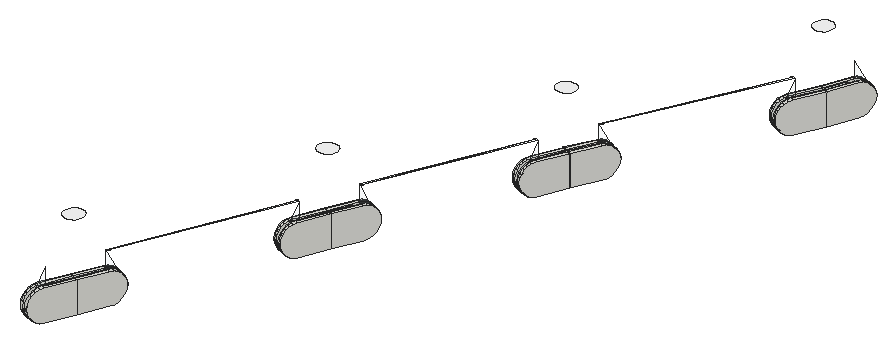
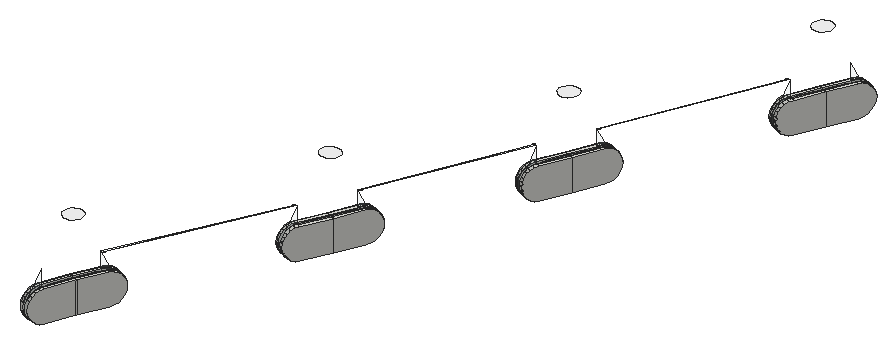
# SketchUp Ruby script. Lengths in inches.
U = 1.inch
M = Sketchup.active_model
def pt(a) = Geom::Point3d.new(a.map { |v| v * U })
def face(e, loops, mat)
  f = e.add_face(loops[0].map { |a| pt(a) })
  loops[1..].each { |l| e.add_face(l.map { |a| pt(a) }).erase! }
  f.material = f.back_material = mat if mat
  f
end
# faces: each face lists its corners as indices into pts; further lists are holes
def faces(e, pts, list, mat = nil) = list.each { |f| face(e, (f[0].is_a?(Array) ? f : [f]).map { |l| l.map { |i| pts[i] } }, mat) }
# xy, xz, yz: faces in a plane at the given z, y or x. An outline is a flat list of corners, or four numbers for a rectangle; further outlines are holes
def ring(l) = l.size == 4 ? [[l[0], l[1]], [l[2], l[1]], [l[2], l[3]], [l[0], l[3]]] : l.each_slice(2).to_a
def flat(e, list, mat, &to3) = list.each { |f| face(e, (f[0].is_a?(Array) ? f : [f]).map { |l| ring(l).map { |u, v| to3.(u, v) } }, mat) }
def xy(e, z, list, mat = nil) = flat(e, list, mat) { |x, y| [x, y, z] }
def xz(e, y, list, mat = nil) = flat(e, list, mat) { |x, z| [x, y, z] }
def yz(e, x, list, mat = nil) = flat(e, list, mat) { |y, z| [x, y, z] }
def lines(e, pts, list) = list.each { |a, b| e.add_line(pt(pts[a]), pt(pts[b])) }
# prism: a flat outline (further loops are holes) pulled along v
def prism(e, loops, v, mat = nil)
  f = face(e, loops, mat); d = Geom::Vector3d.new(v.map { |x| x * U })
  f.pushpull(f.normal.samedirection?(d) ? d.length : -d.length)
end
def box(e, o, s, mat = nil) = prism(e, [[o, [o[0] + s[0], o[1], o[2]], [o[0] + s[0], o[1] + s[1], o[2]], [o[0], o[1] + s[1], o[2]]]], [0, 0, s[2]], mat)
def at(x, y, z, deg = 0) = Geom::Transformation.translation(pt([x, y, z])) * Geom::Transformation.rotation(ORIGIN, Z_AXIS, deg.degrees)
def axes(o, x, y, z) = Geom::Transformation.new([*x, 0, *y, 0, *z, 0, *pt(o).to_a, 1])
def part(name) = M.definitions.add(name)
# library, detail: a bought-in or finely detailed component or shape, given as its bounding box
def library(name, o, s) = part(name).tap { |d| box(d.entities, o, s) }
def detail(e, o, s) = box(e.add_group.entities, o, s)
def put(e, d, t, mat = nil) = e.add_instance(d, t).tap { |i| i.material = mat if mat }
def group(e, t, mat = nil) = e.add_group.tap { |g| g.transformation = t; g.material = mat if mat }.entities
root = M.entities
M.materials.add("Glass_Safety_01").color = [204, 235, 244]
M.materials["Glass_Safety_01"].alpha = 0.1
M.materials.add("[Color_000]").color = [255, 255, 255]
xy(root,351.283,[[864.446,583.7,864.194,583.81,864.292,584.037,864.98,585.615,865.232,585.505],[864.013,583.889,863.761,583.999,864.547,585.803,864.799,585.693,864.112,584.115],[865.232,585.505,864.98,585.615,865.766,587.42,866.018,587.309],[864.799,585.693,864.547,585.803,865.333,587.608,865.585,587.498],[870.556,597.727,870.303,597.837,870.404,598.069,871.089,599.642,871.341,599.53],
  [870.122,597.916,869.87,598.026,870.656,599.83,870.908,599.72,870.224,598.148],[871.341,599.53,871.089,599.642,871.342,599.532],[871.342,599.532,871.089,599.642,871.885,601.441,872.137,601.33],[870.908,599.72,870.656,599.832,871.453,601.633,871.705,601.521],[876.349,610.851,876.097,610.963,876.207,611.21,876.893,612.761,877.142,612.643],
  [875.917,611.043,875.665,611.154,876.462,612.954,876.714,612.843,876.027,611.29],[877.142,612.643,876.893,612.761,876.894,612.763,877.146,612.652,877.144,612.647],[877.146,612.652,876.894,612.763,877.734,614.541,877.983,614.423],[876.715,612.845,876.466,612.963,877.307,614.743,877.556,614.625],[882.822,624.661,882.573,624.779,882.681,625.009,883.414,626.559,883.663,626.441],
  [882.395,624.863,882.145,624.981,882.977,626.738,883.233,626.637,882.503,625.093],[883.672,626.464,883.416,626.565,884.14,628.396,884.396,628.294],[883.233,626.637,882.977,626.738,882.981,626.75,882.986,626.761,883.236,626.643],[883.236,626.643,882.986,626.761,883.7,628.569,883.957,628.468]])
xy(root,351.362,[[864.351,584.171,864.17,584.25,864.799,585.693,864.98,585.615],[864.98,585.615,864.799,585.693,865.428,587.137,865.609,587.059],[870.46,598.198,870.28,598.277,870.908,599.72,870.999,599.681,871.089,599.642],[871.089,599.642,870.999,599.681,870.908,599.72,871.546,601.161,871.726,601.081],[876.257,611.323,876.077,611.403,876.714,612.843,876.804,612.803,876.893,612.761],
  [876.893,612.761,876.804,612.803,876.894,612.763,876.893,612.762],[876.894,612.763,876.804,612.803,876.715,612.845,877.388,614.269,877.566,614.185],[882.741,625.135,882.563,625.219,883.233,626.637,883.325,626.601,883.414,626.559],[883.416,626.565,883.325,626.601,883.236,626.643,883.812,628.102,883.995,628.029],[883.325,626.601,883.233,626.637,883.234,626.64,883.236,626.643]],"Glass_Safety_01")
xy(root,353.33,[[864.351,584.171,864.98,585.615,864.799,585.693,864.17,584.25],[864.98,585.615,865.609,587.059,865.428,587.137,864.799,585.693],[870.46,598.198,871.089,599.642,870.999,599.681,870.908,599.72,870.28,598.277],[871.089,599.642,871.726,601.081,871.546,601.161,870.908,599.72,870.999,599.681],[876.257,611.323,876.893,612.761,876.804,612.803,876.714,612.843,876.077,611.403],
  [876.893,612.761,876.893,612.762,876.894,612.763,876.804,612.803],[876.894,612.763,877.566,614.185,877.388,614.269,876.715,612.845,876.804,612.803],[882.741,625.135,883.414,626.559,883.325,626.601,883.233,626.637,882.563,625.219],[883.416,626.565,883.995,628.029,883.812,628.102,883.236,626.643,883.325,626.601],[883.325,626.601,883.236,626.643,883.234,626.64,883.233,626.637]],"Glass_Safety_01")
xy(root,353.409,[[864.446,583.7,865.232,585.505,864.98,585.615,864.292,584.037,864.194,583.81],[864.013,583.889,864.112,584.115,864.799,585.693,864.547,585.803,863.761,583.999],[865.232,585.505,866.018,587.309,865.766,587.42,864.98,585.615],[864.799,585.693,865.585,587.498,865.333,587.608,864.547,585.803],[870.556,597.727,871.341,599.53,871.089,599.642,870.404,598.069,870.303,597.837],
  [870.122,597.916,870.224,598.148,870.908,599.72,870.656,599.83,869.87,598.026],[871.341,599.53,871.342,599.532,871.089,599.642],[871.342,599.532,872.137,601.33,871.885,601.441,871.089,599.642],[870.908,599.72,871.705,601.521,871.453,601.633,870.656,599.832],[876.349,610.851,877.142,612.643,876.893,612.761,876.207,611.21,876.097,610.963],
  [875.917,611.043,876.027,611.29,876.714,612.843,876.462,612.954,875.665,611.154],[877.142,612.643,877.144,612.647,877.146,612.652,876.894,612.763,876.893,612.761],[877.146,612.652,877.983,614.423,877.734,614.541,876.894,612.763],[876.715,612.845,877.556,614.625,877.307,614.743,876.466,612.963],[882.822,624.661,883.663,626.441,883.414,626.559,882.681,625.009,882.573,624.779],
  [882.395,624.863,882.503,625.093,883.233,626.637,882.977,626.738,882.145,624.981],[883.672,626.464,884.396,628.294,884.14,628.396,883.416,626.565],[883.233,626.637,883.236,626.643,882.986,626.761,882.981,626.75,882.977,626.738],[883.236,626.643,883.957,628.468,883.7,628.569,882.986,626.761]])
xy(root,354.511,[[865.766,587.42,870.224,598.148,865.585,587.498],[865.766,587.42,870.404,598.069,870.224,598.148],[871.885,601.441,876.027,611.29,871.705,601.521],[871.885,601.441,876.207,611.21,876.027,611.29],[877.734,614.541,882.503,625.093,877.556,614.625],
  [877.734,614.541,882.681,625.009,882.503,625.093]],"Glass_Safety_01")
xy(root,357.267,[[864.935,585.026,865.096,585.059,865.243,585.132,865.366,585.242,865.456,585.379,865.508,585.535,865.518,585.699,865.485,585.86,865.411,586.007,865.302,586.13,865.165,586.221,865.009,586.273,864.844,586.282,864.683,586.249,864.536,586.176,864.413,586.066,864.323,585.929,864.271,585.773,864.261,585.609,864.294,585.448,864.368,585.301,864.477,585.178,864.614,585.087,864.77,585.035],[871.044,599.053,871.205,599.086,871.352,599.159,871.475,599.269,871.565,599.406,871.617,599.562,871.627,599.726,871.594,599.887,871.52,600.034,871.411,600.157,871.274,600.248,871.118,600.3,870.954,600.309,870.793,600.276,870.646,600.203,870.523,600.093,870.432,599.956,870.38,599.8,870.37,599.636,870.403,599.475,870.477,599.328,870.586,599.205,870.724,599.114,870.88,599.0625],[876.849,612.175,877.01,612.208,877.157,612.281,877.28,612.391,877.37,612.528,877.422,612.684,877.432,612.848,877.399,613.009,877.325,613.156,877.216,613.279,877.079,613.37,876.923,613.422,876.759,613.431,876.598,613.398,876.451,613.325,876.328,613.215,876.237,613.078,876.185,612.922,876.175,612.758,876.208,612.597,876.282,612.45,876.391,612.327,876.529,612.236,876.685,612.184],[883.37,625.973,883.531,626.006,883.678,626.079,883.801,626.189,883.891,626.326,883.943,626.482,883.953,626.646,883.92,626.807,883.846,626.954,883.737,627.077,883.6,627.168,883.444,627.22,883.28,627.229,883.119,627.196,882.971,627.123,882.849,627.013,882.758,626.876,882.706,626.72,882.696,626.556,882.729,626.395,882.803,626.248,882.912,626.125,883.049,626.034,883.206,625.982]],"[Color_000]")
p = [[865.232,585.505,353.409],[864.446,583.7,353.409],[864.337,583.448,353.373],[864.234,583.213,353.267],[864.146,583.011,353.098],[864.079,582.856,352.877],
  [864.036,582.759,352.621],[864.022,582.725,352.346],[864.036,582.759,352.071],[864.079,582.856,351.815],[864.146,583.011,351.594],[864.234,583.213,351.425],
  [864.337,583.448,351.319],[864.446,583.7,351.283],[865.232,585.505,351.283],[864.013,583.889,351.283],[864.112,584.115,351.283],[864.112,584.115,353.409],
  [864.013,583.889,353.409],[863.903,583.636,353.373],[863.801,583.401,353.267],[863.713,583.199,353.098],[863.646,583.045,352.877],[863.603,582.947,352.621],
  [863.589,582.914,352.346],[863.603,582.947,352.071],[863.646,583.045,351.815],[863.713,583.199,351.594],[863.801,583.401,351.425],[863.903,583.636,351.319],
  [864.292,584.037,353.409],[864.292,584.037,351.283],[864.194,583.81,351.283],[864.084,583.558,351.319],[863.981,583.323,351.425],[863.894,583.121,351.594],
  [863.826,582.966,351.815],[863.784,582.869,352.071],[863.782,582.865,352.098],[864.043,583.463,353.33],[864.084,583.558,353.373],[864.194,583.81,353.409],
  [863.761,583.999,353.409],[864.547,585.803,353.409],[864.547,585.803,351.283],[863.761,583.999,351.283],[863.651,583.746,351.319],[863.548,583.511,351.425],
  [863.46,583.31,351.594],[863.393,583.155,351.815],[863.351,583.057,352.071],[863.336,583.024,352.346],[863.351,583.057,352.621],[863.393,583.155,352.877],
  [863.46,583.31,353.098],[863.548,583.511,353.267],[863.651,583.746,353.373],[864.98,585.615,351.283],[864.98,585.615,353.409],[864.98,585.615,353.33],
  [864.351,584.171,353.33],[864.351,584.171,351.362],[864.98,585.615,351.362],[864.799,585.693,353.409],[864.799,585.693,351.283],[864.799,585.693,351.362],
  [864.17,584.25,351.362],[864.17,584.25,353.33],[864.799,585.693,353.33],[866.018,587.309,353.409],[866.018,587.309,351.283],[866.128,587.562,351.319],
  [866.231,587.797,351.425],[866.319,587.999,351.594],[866.386,588.153,351.815],[866.428,588.251,352.071],[866.443,588.284,352.346],[866.428,588.251,352.621],
  [866.386,588.153,352.877],[866.319,587.999,353.098],[866.231,587.797,353.267],[866.128,587.562,353.373],[865.766,587.42,353.409],[865.766,587.42,351.283],
  [865.609,587.059,351.362],[865.609,587.059,353.33],[865.585,587.498,351.283],[865.585,587.498,353.409],[865.428,587.137,353.33],[865.428,587.137,351.362],
  [865.333,587.608,353.409],[865.442,587.86,353.373],[865.545,588.095,353.267],[865.633,588.297,353.098],[865.7,588.452,352.877],[865.743,588.55,352.621],
  [865.757,588.583,352.346],[865.743,588.55,352.071],[865.7,588.452,351.815],[865.633,588.297,351.594],[865.545,588.095,351.425],[865.442,587.86,351.319],
  [865.333,587.608,351.283],[865.876,587.672,351.319],[865.978,587.907,351.425],[866.066,588.109,351.594],[866.133,588.264,351.815],[866.176,588.361,352.071],
  [866.19,588.394,352.346],[866.176,588.361,352.621],[866.133,588.264,352.877],[866.066,588.109,353.098],[865.978,587.907,353.267],[865.876,587.672,353.373],
  [865.695,587.75,351.319],[865.798,587.985,351.425],[865.885,588.187,351.594],[865.953,588.342,351.815],[865.995,588.439,352.071],[866.01,588.473,352.346],
  [866.003,588.457,352.475],[865.869,588.149,353.13],[865.798,587.985,353.267],[865.695,587.75,353.373],[870.556,597.727,351.283],[871.341,599.53,351.283],
  [871.341,599.53,353.409],[870.556,597.727,353.409],[870.446,597.475,353.373],[870.343,597.24,353.267],[870.255,597.038,353.098],[870.188,596.883,352.877],
  [870.146,596.786,352.621],[870.131,596.752,352.346],[870.146,596.786,352.071],[870.188,596.883,351.815],[870.255,597.038,351.594],[870.343,597.24,351.425],
  [870.446,597.475,351.319],[870.122,597.916,351.283],[870.224,598.148,351.283],[870.224,598.148,353.409],[870.122,597.916,353.409],[870.013,597.663,353.373],
  [869.91,597.428,353.267],[869.822,597.226,353.098],[869.755,597.072,352.877],[869.712,596.974,352.621],[869.698,596.941,352.346],[869.712,596.974,352.071],
  [869.755,597.072,351.815],[869.822,597.226,351.594],[869.91,597.428,351.425],[870.013,597.663,351.319],[870.404,598.069,353.409],[870.404,598.069,351.283],
  [870.303,597.837,351.283],[870.193,597.585,351.319],[870.091,597.35,351.425],[870.003,597.148,351.594],[869.935,596.993,351.815],[869.898,596.906,352.042],
  [870.164,597.519,353.343],[870.193,597.585,353.373],[870.303,597.837,353.409],[869.87,598.026,353.409],[870.656,599.83,353.409],[870.656,599.83,351.283],
  [869.87,598.026,351.283],[869.76,597.773,351.319],[869.658,597.538,351.425],[869.57,597.337,351.594],[869.502,597.182,351.815],[869.46,597.084,352.071],
  [869.445,597.051,352.346],[869.46,597.084,352.621],[869.502,597.182,352.877],[869.57,597.337,353.098],[869.658,597.538,353.267],[869.76,597.773,353.373],
  [870.908,599.72,353.409],[870.908,599.72,351.283],[870.908,599.72,351.362],[870.28,598.277,351.362],[870.28,598.277,353.33],[870.908,599.72,353.33],
  [871.089,599.642,351.283],[871.089,599.642,353.409],[871.089,599.642,353.33],[870.46,598.198,353.33],[870.46,598.198,351.362],[871.089,599.642,351.362],
  [871.342,599.532,353.409],[871.342,599.532,351.283],[872.137,601.33,353.409],[872.137,601.33,351.283],[872.248,601.582,351.319],[872.352,601.816,351.425],
  [872.441,602.017,351.594],[872.51,602.172,351.815],[872.553,602.269,352.071],[872.567,602.302,352.346],[872.553,602.269,352.621],[872.51,602.172,352.877],
  [872.441,602.017,353.098],[872.352,601.816,353.267],[872.248,601.582,353.373],[871.885,601.441,353.409],[871.885,601.441,351.283],[871.726,601.081,351.362],
  [871.726,601.081,353.33],[870.656,599.832,353.409],[870.656,599.832,351.283],[871.705,601.521,351.283],[871.705,601.521,353.409],[871.546,601.161,353.33],
  [871.546,601.161,351.362],[871.453,601.633,353.409],[871.564,601.884,353.373],[871.668,602.119,353.267],[871.757,602.32,353.098],[871.825,602.474,352.877],
  [871.868,602.572,352.621],[871.883,602.605,352.346],[871.868,602.572,352.071],[871.825,602.474,351.815],[871.757,602.32,351.594],[871.668,602.119,351.425],
  [871.564,601.884,351.319],[871.453,601.633,351.283],[871.996,601.693,351.319],[872.1,601.927,351.425],[872.189,602.129,351.594],[872.258,602.283,351.815],
  [872.3,602.38,352.071],[872.315,602.414,352.346],[872.3,602.38,352.621],[872.258,602.283,352.877],[872.189,602.129,353.098],[872.1,601.927,353.267],
  [871.996,601.693,353.373],[871.816,601.773,351.319],[871.92,602.007,351.425],[872.009,602.208,351.594],[872.077,602.363,351.815],[872.12,602.46,352.071],
  [872.132,602.485,352.279],[871.956,602.088,353.199],[871.92,602.007,353.267],[871.816,601.773,353.373],[876.349,610.851,351.283],[877.142,612.643,351.283],
  [877.142,612.643,353.409],[876.349,610.851,353.409],[876.238,610.6,353.373],[876.134,610.365,353.267],[876.045,610.164,353.098],[875.977,610.01,352.877],
  [875.934,609.912,352.621],[875.919,609.879,352.346],[875.934,609.912,352.071],[875.977,610.01,351.814],[876.045,610.164,351.594],[876.134,610.365,351.425],
  [876.238,610.6,351.319],[876.207,611.21,353.409],[876.893,612.761,353.409],[876.893,612.761,353.33],[876.893,612.761,351.362],[876.893,612.761,351.283],
  [876.207,611.21,351.283],[876.097,610.963,351.283],[875.986,610.711,351.319],[875.882,610.477,351.425],[875.793,610.276,351.594],[875.725,610.121,351.814],
  [875.709,610.086,351.908],[875.682,610.024,352.071],[875.667,609.991,352.346],[875.682,610.024,352.621],[875.725,610.121,352.877],[875.793,610.276,353.098],
  [875.882,610.477,353.267],[875.986,610.711,353.373],[875.989,610.719,353.374],[876.097,610.963,353.409],[875.917,611.043,351.283],[876.027,611.29,351.283],
  [876.027,611.29,353.409],[875.917,611.043,353.409],[875.806,610.791,353.373],[875.702,610.557,353.267],[875.613,610.355,353.098],[875.545,610.201,352.877],
  [875.502,610.104,352.621],[875.487,610.07,352.346],[875.502,610.104,352.071],[875.545,610.201,351.814],[875.613,610.355,351.594],[875.702,610.557,351.425],
  [875.806,610.791,351.319],[875.665,611.154,353.409],[876.462,612.954,353.409],[876.462,612.954,351.283],[875.665,611.154,351.283],[875.554,610.902,351.319],
  [875.45,610.668,351.425],[875.361,610.467,351.594],[875.293,610.312,351.814],[875.25,610.215,352.071],[875.235,610.182,352.346],[875.25,610.215,352.621],
  [875.293,610.312,352.877],[875.361,610.467,353.098],[875.45,610.668,353.267],[875.554,610.902,353.373],[876.714,612.843,353.409],[876.714,612.843,351.283],
  [876.714,612.843,351.362],[876.077,611.403,351.362],[876.077,611.403,353.33],[876.714,612.843,353.33],[877.144,612.647,353.409],[877.144,612.647,351.283],
  [877.146,612.652,351.283],[877.146,612.652,353.409],[877.983,614.423,351.283],[878.101,614.672,351.319],[878.21,614.903,351.425],[878.304,615.103,351.594],
  [878.376,615.255,351.814],[878.422,615.351,352.071],[878.437,615.384,352.346],[878.422,615.351,352.621],[878.376,615.255,352.877],[878.304,615.103,353.098],
  [878.21,614.903,353.267],[878.101,614.672,353.373],[877.983,614.423,353.409],[876.894,612.763,351.283],[876.894,612.763,351.362],[876.894,612.763,353.33],
  [876.894,612.763,353.409],[876.715,612.845,351.283],[876.715,612.845,351.362],[876.715,612.845,353.33],[876.715,612.845,353.409],[876.466,612.963,353.409],
  [876.466,612.963,351.283],[877.556,614.625,351.283],[877.556,614.625,353.409],[877.388,614.269,353.33],[877.388,614.269,351.362],[877.734,614.541,353.409],
  [877.851,614.789,353.373],[877.961,615.021,353.267],[878.055,615.22,353.098],[878.127,615.373,352.877],[878.173,615.469,352.621],[878.188,615.502,352.346],
  [878.173,615.469,352.071],[878.127,615.373,351.814],[878.055,615.22,351.594],[877.961,615.021,351.425],[877.851,614.789,351.319],[877.734,614.541,351.283],
  [877.307,614.743,353.409],[877.424,614.991,353.373],[877.534,615.223,353.267],[877.628,615.422,353.098],[877.7,615.575,352.877],[877.745,615.671,352.621],
  [877.761,615.704,352.346],[877.745,615.671,352.071],[877.7,615.575,351.814],[877.628,615.422,351.594],[877.534,615.223,351.425],[877.424,614.991,351.319],
  [877.307,614.743,351.283],[877.673,614.874,351.319],[877.783,615.105,351.425],[877.877,615.304,351.594],[877.949,615.457,351.814],[877.995,615.553,352.071],
  [878.01,615.586,352.346],[878.003,615.572,352.466],[877.857,615.263,353.133],[877.783,615.105,353.267],[877.673,614.874,353.373],[883.663,626.441,353.409],
  [882.822,624.661,353.409],[882.704,624.413,353.373],[882.595,624.181,353.267],[882.501,623.982,353.098],[882.428,623.829,352.877],[882.383,623.733,352.621],
  [882.367,623.7,352.346],[882.383,623.733,352.071],[882.428,623.829,351.814],[882.501,623.982,351.594],[882.595,624.181,351.425],[882.704,624.413,351.319],
  [882.822,624.661,351.283],[883.663,626.441,351.283],[882.503,625.093,353.409],[882.503,625.093,351.283],[882.395,624.863,351.283],[882.277,624.615,351.319],
  [882.167,624.383,351.425],[882.073,624.184,351.594],[882.001,624.031,351.814],[881.956,623.935,352.071],[881.94,623.902,352.346],[881.956,623.935,352.621],
  [882.001,624.031,352.877],[882.073,624.184,353.098],[882.167,624.383,353.267],[882.277,624.615,353.373],[882.395,624.863,353.409],[883.233,626.637,351.283],
  [883.233,626.637,351.362],[883.233,626.637,353.33],[883.233,626.637,353.409],[882.681,625.009,353.409],[882.681,625.009,351.283],[882.573,624.779,351.283],
  [882.455,624.53,351.319],[882.345,624.299,351.425],[882.251,624.1,351.594],[882.179,623.947,351.814],[882.14,623.863,352.037],[882.426,624.469,353.344],
  [882.455,624.53,353.373],[882.573,624.779,353.409],[882.145,624.981,353.409],[882.977,626.738,353.409],[882.977,626.738,351.283],[882.145,624.981,351.283],
  [882.028,624.732,351.319],[881.918,624.501,351.425],[881.824,624.301,351.594],[881.752,624.149,351.814],[881.707,624.053,352.071],[881.691,624.02,352.346],
  [881.707,624.053,352.621],[881.752,624.149,352.877],[881.824,624.301,353.098],[881.918,624.501,353.267],[882.028,624.732,353.373],[883.414,626.559,351.283],
  [883.414,626.559,353.409],[883.414,626.559,353.33],[882.741,625.135,353.33],[882.741,625.135,351.362],[883.414,626.559,351.362],[883.416,626.565,351.362],
  [883.416,626.565,351.283],[883.672,626.464,351.283],[883.672,626.464,353.409],[883.416,626.565,353.409],[883.416,626.565,353.33],[884.396,628.294,353.409],
  [884.396,628.294,351.283],[884.497,628.55,351.319],[884.591,628.789,351.425],[884.672,628.993,351.594],[884.734,629.15,351.814],[884.773,629.249,352.071],
  [884.787,629.283,352.346],[884.773,629.249,352.621],[884.734,629.15,352.877],[884.672,628.993,353.098],[884.591,628.789,353.267],[884.497,628.55,353.373],
  [883.236,626.643,351.362],[883.236,626.643,351.283],[882.986,626.761,351.283],[882.986,626.761,353.409],[883.236,626.643,353.409],[883.236,626.643,353.33],
  [883.957,628.468,351.283],[884.058,628.724,351.319],[884.152,628.962,351.425],[884.233,629.167,351.594],[884.295,629.324,351.814],[884.334,629.423,352.071],
  [884.347,629.456,352.346],[884.334,629.423,352.621],[884.329,629.411,352.653],[884.295,629.324,352.877],[884.257,629.229,353.01],[884.233,629.167,353.098],
  [884.152,628.962,353.267],[884.058,628.724,353.373],[883.957,628.468,353.409],[884.14,628.396,353.409],[884.14,628.396,351.283],[883.995,628.029,351.362],
  [883.995,628.029,353.33],[882.981,626.75,351.283],[882.981,626.75,353.409],[883.7,628.569,353.409],[883.801,628.825,353.373],[883.896,629.063,353.267],
  [883.977,629.268,353.098],[884.039,629.425,352.877],[884.078,629.524,352.621],[884.091,629.558,352.346],[884.078,629.524,352.071],[884.039,629.425,351.814],
  [883.977,629.268,351.594],[883.896,629.063,351.425],[883.801,628.825,351.319],[883.7,628.569,351.283],[884.241,628.651,351.319],[884.335,628.89,351.425],
  [884.416,629.095,351.594],[884.478,629.252,351.814],[884.517,629.35,352.071],[884.53,629.384,352.346],[884.517,629.35,352.621],[884.478,629.252,352.877],
  [884.416,629.095,353.098],[884.335,628.89,353.267],[884.241,628.651,353.373],[870.999,599.681,351.362],[870.999,599.681,353.33],[876.257,611.323,351.362],
  [876.257,611.323,353.33],[876.804,612.803,353.33],[876.804,612.803,351.362],[876.893,612.762,351.362],[876.893,612.762,353.33],[877.566,614.185,353.33],
  [877.566,614.185,351.362],[882.563,625.219,353.33],[882.563,625.219,351.362],[883.325,626.601,351.362],[883.325,626.601,353.33],[883.234,626.64,353.33],
  [883.234,626.64,351.362],[883.812,628.102,351.362],[883.812,628.102,353.33],[869.893,596.896,352.071],[882.134,623.851,352.071],[869.878,596.862,352.346],
  [869.893,596.896,352.621],[869.935,596.993,352.877],[870.003,597.148,353.098],[870.091,597.35,353.267],[882.118,623.818,352.346],[882.134,623.851,352.621],
  [882.179,623.947,352.877],[882.251,624.1,353.098],[882.345,624.299,353.267],[863.769,582.835,352.346],[863.784,582.869,352.621],[863.826,582.966,352.877],
  [863.894,583.121,353.098],[863.981,583.323,353.267],[872.135,602.493,352.346],[865.995,588.439,352.621],[872.009,602.208,353.098],[872.077,602.363,352.877],
  [872.12,602.46,352.621],[877.995,615.553,352.621],[865.885,588.187,353.098],[865.953,588.342,352.877],[877.877,615.304,353.098],[877.949,615.457,352.877],
  [883.957,628.468,354.511],[865.585,587.498,354.511],[877.556,614.625,354.511],[871.705,601.521,354.511],[864.292,584.037,354.511],[870.404,598.069,354.511],
  [882.681,625.009,354.511],[876.207,611.21,354.511]]
faces(root,p,[[0,1,2,3,4,5,6,7,8,9,10,11,12,13,14],[15,16,17,18,19,20,21,22,23,24,25,26,27,28,29],[42,43,44,45,46,47,48,49,50,51,52,53,54,55,56],[34,33,12,11],[29,28,47,46],[33,32,13,12],[15,29,46,45],[57,31,30,58,59,60,61,62],
  [63,17,16,64,65,66,67,68],[57,62,59,58,0,14],[69,0,14,70,71,72,73,74,75,76,77,78,79,80,81],[58,82,83,57,62,84,85,59],[65,64,44,43,63,68],[64,86,87,63,68,88,89,65],[43,90,91,92,93,94,95,96,97,98,99,100,101,102,44],[83,103,71,70],
  [114,86,102,101],[103,104,72,71],[115,114,101,100],[124,125,126,127,128,129,130,131,132,133,134,135,136,137,138],[139,140,141,142,143,144,145,146,147,148,149,150,151,152,153],[165,166,167,168,169,170,171,172,173,174,175,176,177,178,179],[158,157,138,137],[153,152,170,169],
  [157,156,124,138],[139,153,169,168],[180,141,140,181,182,183,184,185],[186,155,154,187,188,189,190,191],[191,186,125,126,187,188],[186,191,188,187,192,193],[125,193,192,126],[194,192,193,195,196,197,198,199,200,201,202,203,204,205,206],
  [187,207,208,186,191,209,210,188],[182,181,167,166,180,185],[181,182,185,180,211,212],[181,213,214,180,185,215,216,182],[211,217,218,219,220,221,222,223,224,225,226,227,228,229,212],[208,230,196,195],[241,213,229,228],[230,231,197,196],
  [242,241,228,227],[250,251,252,253,254,255,256,257,258,259,260,261,262,263,264],[265,266,267,268,269,270,271,272,273,274,275,276,277,278,279,280,281,282,283,284,285],[286,287,288,289,290,291,292,293,294,295,296,297,298,299,300],[301,302,303,304,305,306,307,308,309,310,311,312,313,314,315],[273,272,264,263],[300,299,306,305],[272,271,250,264],
  [286,300,305,304],[316,288,287,317,318,319,320,321],[268,269,251,252,266,267],[322,252,251,323,324,325],[322,252,251,323,324,326,327,328,329,330,331,332,333,334,335,336,337,338,325],[339,340,341,342,325,324],[318,317,303,302,316,321],[343,344,345,346,347,348],
  [343,349,350,346,345,351,352,344],[339,269,268,267,266,342,341,340],[266,342,353,354,355,356,357,358,359,360,361,362,363,364,365,339,269,268,267],[347,366,367,368,369,370,371,372,373,374,375,376,377,378,348],[365,364,327,326],[379,349,378,377],[364,363,328,327],[380,379,377,376],
  [389,390,391,392,393,394,395,396,397,398,399,400,401,402,403],[406,405,419,420,421,422,404,418,417,416,415,414,413,412,411,410,409,408,407],[434,435,436,437,438,439,440,441,442,443,444,445,446,447,448],[427,426,401,400],[407,408,439,438],[426,425,402,401],[406,407,438,437],[449,424,423,450,451,452,453,454],
  [449,454,451,450,389,403],[455,456,457,458,459,460],[461,458,457,462,463,464,465,466,467,468,469,470,471,472,473],[419,420,421,422,435,436],[474,475,476,477,478,479],[478,422,421,420,419,475,474,479],[478,422,421,420,419,475,480,481,482,483,484,485,486,487,488,489,490,491,492,493,494],[459,495,496,456,455,497,498,460],
  [499,436,435,500,477,476],[435,500,477,501,502,503,504,505,506,507,508,509,510,511,512,513,476,499,436],[496,514,463,462],[481,480,513,512],[514,515,464,463],[482,481,512,511],[35,34,11,10],[28,27,48,47],
  [104,105,73,72],[116,115,100,99],[159,158,137,136],[152,151,171,170],[231,232,198,197],[243,242,227,226],[274,273,263,262],[299,298,307,306],
  [363,362,329,328],[381,380,376,375],[428,427,400,399],[408,409,440,439],[515,516,465,464],[483,482,511,510],[36,35,10,9],[27,26,49,48],
  [105,106,74,73],[117,116,99,98],[160,159,136,135],[151,150,172,171],[232,233,199,198],[244,243,226,225],[275,274,262,261],[298,297,308,307],
  [362,361,330,329],[382,381,375,374],[429,428,399,398],[409,410,441,440],[516,517,466,465],[26,25,50,49],[106,107,75,74],[118,117,98,97],
  [543,161,160,135,134],[150,149,173,172],[233,234,200,199],[245,244,225,224],[277,276,275,261,260],[297,296,309,308],[361,360,331,330],[383,382,374,373],
  [544,430,429,398,397],[410,411,442,441],[517,518,467,466],[161,543,545,546,547,548,549,162],[430,544,550,551,552,553,554,431],[38,555,556,557,558,559,39],[107,108,76,75],[119,118,97,96],
  [545,543,134,133],[149,148,174,173],[234,235,201,200],[560,246,245,224,223],[278,277,260,259],[296,295,310,309],[360,359,332,331],[384,383,373,372],
  [550,544,397,396],[411,412,443,442],[108,109,77,76],[561,120,119,96,95],[546,545,133,132],[148,147,175,174],[235,236,202,201],[564,560,223,222],
  [279,278,259,258],[295,294,311,310],[359,358,333,332],[565,385,384,372,371],[551,550,396,395],[412,413,444,443],[23,22,53,52],[109,110,78,77],
  [567,561,95,94],[547,546,132,131],[147,146,176,175],[236,237,203,202],[563,564,222,221],[280,279,258,257],[294,293,312,311],[358,357,334,333],
  [569,565,371,370],[552,551,395,394],[413,414,445,444],[520,521,470,469],[22,21,54,53],[110,111,79,78],[566,567,94,93],[548,547,131,130],
  [146,145,177,176],[237,238,204,203],[562,563,221,220],[281,280,257,256],[293,292,313,312],[357,356,335,334],[568,569,370,369],[553,552,394,393],
  [414,415,446,445],[521,522,471,470],[491,490,489,505,504],[559,558,4,3],[21,20,55,54],[111,112,80,79],[122,121,566,93,92],[549,548,130,129],
  [145,144,178,177],[238,239,205,204],[248,247,562,220,219],[282,281,256,255],[292,291,314,313],[356,355,336,335],[387,386,568,369,368],[554,553,393,392],
  [415,416,447,446],[522,523,472,471],[492,491,504,503],[40,39,559,3,2],[20,19,56,55],[112,113,81,80],[123,122,92,91],[163,162,549,129,128],
  [144,143,179,178],[239,240,206,205],[249,248,219,218],[283,282,255,254],[291,290,315,314],[355,354,337,336],[388,387,368,367],[432,431,554,392,391],
  [416,417,448,447],[523,524,473,472],[493,492,503,502],[41,40,2,1],[19,18,42,56],[113,82,69,81],[87,123,91,90],[164,163,128,127],
  [143,142,165,179],[240,207,194,206],[214,249,218,217],[285,284,283,254,253],[290,289,301,315],[354,353,338,337],[350,388,367,366],[433,432,391,390],
  [417,418,434,448],[524,495,461,473],[494,493,502,501]])
faces(root,p,[[30,31,32,33,34,35,36,37,38,39,40,41],[82,83,103,104,105,106,107,108,109,110,111,112,113],[87,86,114,115,116,117,118,119,120,121,122,123],[154,155,156,157,158,159,160,161,162,163,164],[207,208,230,231,232,233,234,235,236,237,238,239,240],[214,213,241,242,243,244,245,246,247,248,249],[270,265,285,284,276,275,274,273,272,271],[353,365,364,363,362,361,360,359,358,357,356,355,354],
  [350,349,379,380,381,382,383,384,385,386,387,388],[404,405,406,407,408,409,410,411,412,413,414,415,416,417,418],[423,424,425,426,427,428,429,430,431,432,433],[495,496,514,515,516,517,518,519,520,521,522,523,524],[480,494,493,492,491,490,488,487,486,485,484,483,482,481],[67,66,61,60],[68,67,66,65],[60,59,62,61],
  [68,59,62,65],[59,85,84,62],[88,68,65,89],[85,84,89,88],[184,183,190,189],[189,188,191,190],[185,184,183,182],[191,525,526,188],
  [188,210,209,191],[185,526,525,182],[215,185,182,216],[215,210,209,216],[320,319,527,528],[527,268,267,528],[321,320,319,318],[321,529,530,318],
  [530,529,345,344],[351,345,344,352],[529,530,268,267],[340,530,529,341],[531,340,341,532,267,268],[533,341,340,534],[351,533,534,352],[535,536,453,452],
  [452,451,454,453],[535,421,420,536],[537,538,421,420],[479,538,537,474],[539,479,474,540,420,421],[541,474,479,542],[454,537,538,451],[538,537,455,460],
  [460,498,497,455],[497,541,542,498],[276,284,283,282,281,280,279,278,277],[246,247,562,563,564,560],[120,121,566,567,561],[385,386,568,569,565],[570,490,491,492,493,494],[571,121,122,123,87],
  [572,386,387,388,350],[573,247,248,249,214],[574,39,40,41,30],[575,162,163,164,154],[576,431,432,433,423],[577,284,285,265]],"Glass_Safety_01")
